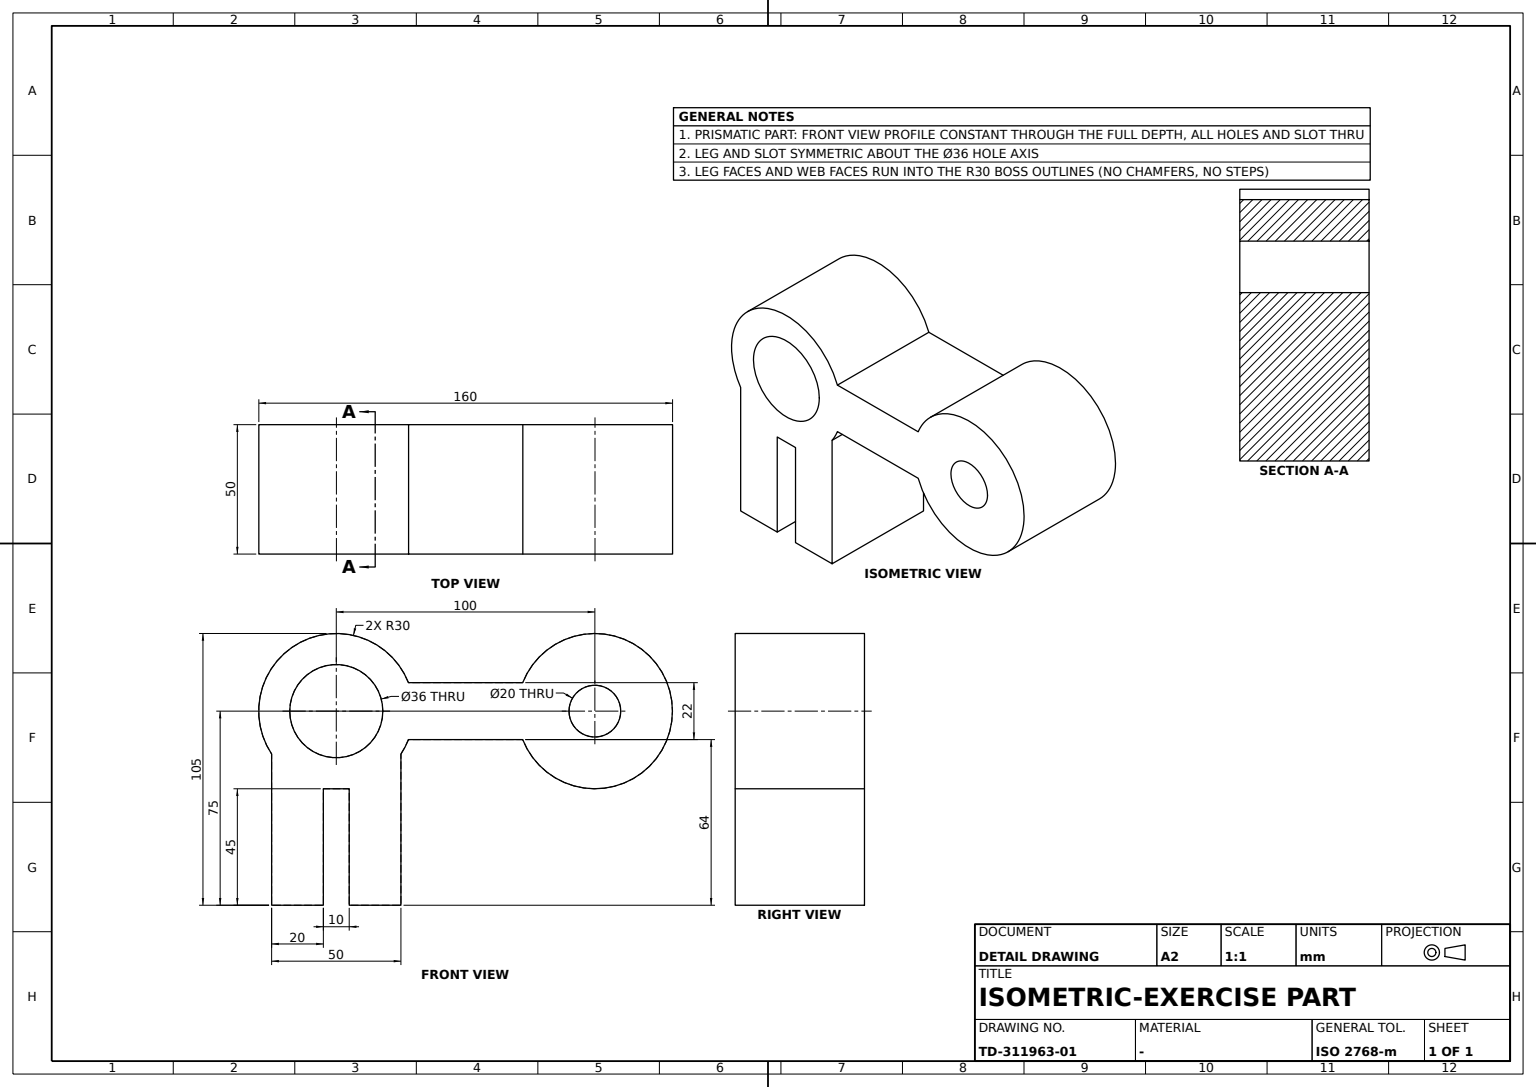
ISO-10303-21;
HEADER;
FILE_DESCRIPTION((''),'2;1');
FILE_NAME('','',(''),(''),'','','');
FILE_SCHEMA(('AUTOMOTIVE_DESIGN'));
ENDSEC;
DATA;
#1=APPLICATION_CONTEXT('');
#2=PRODUCT_CONTEXT('',#1,'mechanical');
#3=PRODUCT('','','',(#2));
#4=PRODUCT_DEFINITION_FORMATION('','',#3);
#5=PRODUCT_DEFINITION_CONTEXT('',#1,'design');
#6=PRODUCT_DEFINITION('','',#4,#5);
#7=PRODUCT_DEFINITION_SHAPE('','',#6);
#8=(LENGTH_UNIT()NAMED_UNIT(*)SI_UNIT(.MILLI.,.METRE.));
#9=(NAMED_UNIT(*)PLANE_ANGLE_UNIT()SI_UNIT($,.RADIAN.));
#10=(NAMED_UNIT(*)SI_UNIT($,.STERADIAN.)SOLID_ANGLE_UNIT());
#11=UNCERTAINTY_MEASURE_WITH_UNIT(LENGTH_MEASURE(1.E-05),#8,'distance_accuracy_value','');
#12=(GEOMETRIC_REPRESENTATION_CONTEXT(3)GLOBAL_UNCERTAINTY_ASSIGNED_CONTEXT((#11))GLOBAL_UNIT_ASSIGNED_CONTEXT((#8,#9,#10))REPRESENTATION_CONTEXT('',''));
#13=CARTESIAN_POINT('',(-25.,-25.,-16.583124));
#14=VERTEX_POINT('',#13);
#15=CARTESIAN_POINT('',(25.,-25.,-16.583124));
#16=VERTEX_POINT('',#15);
#17=CARTESIAN_POINT('',(0.,-25.,-16.583124));
#18=DIRECTION('',(1.,0.,0.));
#19=VECTOR('',#18,1000.);
#20=LINE('',#17,#19);
#21=EDGE_CURVE('',#14,#16,#20,.T.);
#22=ORIENTED_EDGE('',*,*,#21,.T.);
#23=CARTESIAN_POINT('',(25.,27.910571,11.));
#24=VERTEX_POINT('',#23);
#25=CARTESIAN_POINT('',(25.,0.,0.));
#26=DIRECTION('',(0.,1.,0.));
#27=AXIS2_PLACEMENT_3D('',#25,#18,#26);
#28=CIRCLE('',#27,30.);
#29=EDGE_CURVE('',#24,#16,#28,.T.);
#30=ORIENTED_EDGE('',*,*,#29,.F.);
#31=CARTESIAN_POINT('',(-25.,27.910571,11.));
#32=VERTEX_POINT('',#31);
#33=CARTESIAN_POINT('',(0.,27.910571,11.));
#34=LINE('',#33,#19);
#35=EDGE_CURVE('',#32,#24,#34,.T.);
#36=ORIENTED_EDGE('',*,*,#35,.F.);
#37=CARTESIAN_POINT('',(-25.,0.,0.));
#38=AXIS2_PLACEMENT_3D('',#37,#18,#26);
#39=CIRCLE('',#38,30.);
#40=EDGE_CURVE('',#32,#14,#39,.T.);
#41=ORIENTED_EDGE('',*,*,#40,.T.);
#42=EDGE_LOOP('',(#22,#30,#36,#41));
#43=FACE_OUTER_BOUND('',#42,.T.);
#44=CARTESIAN_POINT('',(0.,0.,0.));
#45=DIRECTION('',(-1.,0.,0.));
#46=AXIS2_PLACEMENT_3D('',#44,#45,#26);
#47=CYLINDRICAL_SURFACE('',#46,30.);
#48=ADVANCED_FACE('',(#43),#47,.T.);
#49=CARTESIAN_POINT('',(-25.,-25.,-75.));
#50=VERTEX_POINT('',#49);
#51=CARTESIAN_POINT('',(25.,-25.,-75.));
#52=VERTEX_POINT('',#51);
#53=CARTESIAN_POINT('',(0.,-25.,-75.));
#54=LINE('',#53,#19);
#55=EDGE_CURVE('',#50,#52,#54,.T.);
#56=ORIENTED_EDGE('',*,*,#55,.F.);
#57=CARTESIAN_POINT('',(-25.,-5.,-75.));
#58=VERTEX_POINT('',#57);
#59=CARTESIAN_POINT('',(-25.,-15.,-75.));
#60=VECTOR('',#26,1000.);
#61=LINE('',#59,#60);
#62=EDGE_CURVE('',#50,#58,#61,.T.);
#63=ORIENTED_EDGE('',*,*,#62,.T.);
#64=CARTESIAN_POINT('',(25.,-5.,-75.));
#65=VERTEX_POINT('',#64);
#66=CARTESIAN_POINT('',(0.,-5.,-75.));
#67=LINE('',#66,#19);
#68=EDGE_CURVE('',#58,#65,#67,.T.);
#69=ORIENTED_EDGE('',*,*,#68,.T.);
#70=CARTESIAN_POINT('',(25.,-15.,-75.));
#71=LINE('',#70,#60);
#72=EDGE_CURVE('',#52,#65,#71,.T.);
#73=ORIENTED_EDGE('',*,*,#72,.F.);
#74=EDGE_LOOP('',(#56,#63,#69,#73));
#75=FACE_OUTER_BOUND('',#74,.T.);
#76=DIRECTION('',(0.,0.,-1.));
#77=AXIS2_PLACEMENT_3D('',#53,#76,#26);
#78=PLANE('',#77);
#79=ADVANCED_FACE('',(#75),#78,.T.);
#80=CARTESIAN_POINT('',(25.,25.,-75.));
#81=VERTEX_POINT('',#80);
#82=CARTESIAN_POINT('',(25.,25.,-16.583124));
#83=VERTEX_POINT('',#82);
#84=CARTESIAN_POINT('',(25.,25.,-45.791562));
#85=DIRECTION('',(0.,0.,1.));
#86=VECTOR('',#85,1000.);
#87=LINE('',#84,#86);
#88=EDGE_CURVE('',#81,#83,#87,.T.);
#89=ORIENTED_EDGE('',*,*,#88,.F.);
#90=CARTESIAN_POINT('',(-25.,25.,-75.));
#91=VERTEX_POINT('',#90);
#92=CARTESIAN_POINT('',(0.,25.,-75.));
#93=LINE('',#92,#19);
#94=EDGE_CURVE('',#91,#81,#93,.T.);
#95=ORIENTED_EDGE('',*,*,#94,.F.);
#96=CARTESIAN_POINT('',(-25.,25.,-16.583124));
#97=VERTEX_POINT('',#96);
#98=CARTESIAN_POINT('',(-25.,25.,-45.791562));
#99=LINE('',#98,#86);
#100=EDGE_CURVE('',#91,#97,#99,.T.);
#101=ORIENTED_EDGE('',*,*,#100,.T.);
#102=CARTESIAN_POINT('',(0.,25.,-16.583124));
#103=LINE('',#102,#19);
#104=EDGE_CURVE('',#97,#83,#103,.T.);
#105=ORIENTED_EDGE('',*,*,#104,.T.);
#106=EDGE_LOOP('',(#89,#95,#101,#105));
#107=FACE_OUTER_BOUND('',#106,.T.);
#108=AXIS2_PLACEMENT_3D('',#92,#26,#85);
#109=PLANE('',#108);
#110=ADVANCED_FACE('',(#107),#109,.T.);
#111=CARTESIAN_POINT('',(-25.,110.,0.));
#112=VERTEX_POINT('',#111);
#113=CARTESIAN_POINT('',(25.,110.,0.));
#114=VERTEX_POINT('',#113);
#115=CARTESIAN_POINT('',(0.,110.,0.));
#116=LINE('',#115,#19);
#117=EDGE_CURVE('',#112,#114,#116,.T.);
#118=ORIENTED_EDGE('',*,*,#117,.T.);
#119=CARTESIAN_POINT('',(25.,90.,0.));
#120=VERTEX_POINT('',#119);
#121=CARTESIAN_POINT('',(25.,100.,0.));
#122=AXIS2_PLACEMENT_3D('',#121,#18,#26);
#123=CIRCLE('',#122,10.);
#124=EDGE_CURVE('',#114,#120,#123,.T.);
#125=ORIENTED_EDGE('',*,*,#124,.T.);
#126=CARTESIAN_POINT('',(-25.,90.,0.));
#127=VERTEX_POINT('',#126);
#128=CARTESIAN_POINT('',(0.,90.,0.));
#129=LINE('',#128,#19);
#130=EDGE_CURVE('',#127,#120,#129,.T.);
#131=ORIENTED_EDGE('',*,*,#130,.F.);
#132=CARTESIAN_POINT('',(-25.,100.,0.));
#133=AXIS2_PLACEMENT_3D('',#132,#18,#26);
#134=CIRCLE('',#133,10.);
#135=EDGE_CURVE('',#112,#127,#134,.T.);
#136=ORIENTED_EDGE('',*,*,#135,.F.);
#137=EDGE_LOOP('',(#118,#125,#131,#136));
#138=FACE_OUTER_BOUND('',#137,.T.);
#139=CARTESIAN_POINT('',(0.,100.,0.));
#140=AXIS2_PLACEMENT_3D('',#139,#45,#26);
#141=CYLINDRICAL_SURFACE('',#140,10.);
#142=ADVANCED_FACE('',(#138),#141,.F.);
#143=CARTESIAN_POINT('',(-25.,27.910571,-11.));
#144=VERTEX_POINT('',#143);
#145=CARTESIAN_POINT('',(25.,27.910571,-11.));
#146=VERTEX_POINT('',#145);
#147=CARTESIAN_POINT('',(0.,27.910571,-11.));
#148=LINE('',#147,#19);
#149=EDGE_CURVE('',#144,#146,#148,.T.);
#150=ORIENTED_EDGE('',*,*,#149,.T.);
#151=EDGE_CURVE('',#83,#146,#28,.T.);
#152=ORIENTED_EDGE('',*,*,#151,.F.);
#153=ORIENTED_EDGE('',*,*,#104,.F.);
#154=EDGE_CURVE('',#97,#144,#39,.T.);
#155=ORIENTED_EDGE('',*,*,#154,.T.);
#156=EDGE_LOOP('',(#150,#152,#153,#155));
#157=FACE_OUTER_BOUND('',#156,.T.);
#158=ADVANCED_FACE('',(#157),#47,.T.);
#159=CARTESIAN_POINT('',(25.,72.089429,11.));
#160=VERTEX_POINT('',#159);
#161=CARTESIAN_POINT('',(25.,50.,11.));
#162=DIRECTION('',(0.,-1.,0.));
#163=VECTOR('',#162,1000.);
#164=LINE('',#161,#163);
#165=EDGE_CURVE('',#160,#24,#164,.T.);
#166=ORIENTED_EDGE('',*,*,#165,.F.);
#167=CARTESIAN_POINT('',(-25.,72.089429,11.));
#168=VERTEX_POINT('',#167);
#169=CARTESIAN_POINT('',(0.,72.089429,11.));
#170=LINE('',#169,#19);
#171=EDGE_CURVE('',#168,#160,#170,.T.);
#172=ORIENTED_EDGE('',*,*,#171,.F.);
#173=CARTESIAN_POINT('',(-25.,50.,11.));
#174=LINE('',#173,#163);
#175=EDGE_CURVE('',#168,#32,#174,.T.);
#176=ORIENTED_EDGE('',*,*,#175,.T.);
#177=ORIENTED_EDGE('',*,*,#35,.T.);
#178=EDGE_LOOP('',(#166,#172,#176,#177));
#179=FACE_OUTER_BOUND('',#178,.T.);
#180=AXIS2_PLACEMENT_3D('',#33,#76,#26);
#181=PLANE('',#180);
#182=ADVANCED_FACE('',(#179),#181,.F.);
#183=CARTESIAN_POINT('',(-25.,-5.,-30.));
#184=VERTEX_POINT('',#183);
#185=CARTESIAN_POINT('',(-25.,-5.,-52.5));
#186=LINE('',#185,#86);
#187=EDGE_CURVE('',#58,#184,#186,.T.);
#188=ORIENTED_EDGE('',*,*,#187,.T.);
#189=CARTESIAN_POINT('',(25.,-5.,-30.));
#190=VERTEX_POINT('',#189);
#191=CARTESIAN_POINT('',(0.,-5.,-30.));
#192=LINE('',#191,#19);
#193=EDGE_CURVE('',#184,#190,#192,.T.);
#194=ORIENTED_EDGE('',*,*,#193,.T.);
#195=CARTESIAN_POINT('',(25.,-5.,-52.5));
#196=LINE('',#195,#86);
#197=EDGE_CURVE('',#65,#190,#196,.T.);
#198=ORIENTED_EDGE('',*,*,#197,.F.);
#199=ORIENTED_EDGE('',*,*,#68,.F.);
#200=EDGE_LOOP('',(#188,#194,#198,#199));
#201=FACE_OUTER_BOUND('',#200,.T.);
#202=AXIS2_PLACEMENT_3D('',#191,#162,#76);
#203=PLANE('',#202);
#204=ADVANCED_FACE('',(#201),#203,.F.);
#205=CARTESIAN_POINT('',(-25.,72.089429,-11.));
#206=VERTEX_POINT('',#205);
#207=CARTESIAN_POINT('',(-25.,50.,-11.));
#208=LINE('',#207,#60);
#209=EDGE_CURVE('',#144,#206,#208,.T.);
#210=ORIENTED_EDGE('',*,*,#209,.T.);
#211=CARTESIAN_POINT('',(25.,72.089429,-11.));
#212=VERTEX_POINT('',#211);
#213=CARTESIAN_POINT('',(0.,72.089429,-11.));
#214=LINE('',#213,#19);
#215=EDGE_CURVE('',#206,#212,#214,.T.);
#216=ORIENTED_EDGE('',*,*,#215,.T.);
#217=CARTESIAN_POINT('',(25.,50.,-11.));
#218=LINE('',#217,#60);
#219=EDGE_CURVE('',#146,#212,#218,.T.);
#220=ORIENTED_EDGE('',*,*,#219,.F.);
#221=ORIENTED_EDGE('',*,*,#149,.F.);
#222=EDGE_LOOP('',(#210,#216,#220,#221));
#223=FACE_OUTER_BOUND('',#222,.T.);
#224=AXIS2_PLACEMENT_3D('',#147,#76,#26);
#225=PLANE('',#224);
#226=ADVANCED_FACE('',(#223),#225,.T.);
#227=ORIENTED_EDGE('',*,*,#209,.F.);
#228=ORIENTED_EDGE('',*,*,#154,.F.);
#229=ORIENTED_EDGE('',*,*,#100,.F.);
#230=CARTESIAN_POINT('',(-25.,5.,-75.));
#231=VERTEX_POINT('',#230);
#232=CARTESIAN_POINT('',(-25.,15.,-75.));
#233=LINE('',#232,#60);
#234=EDGE_CURVE('',#231,#91,#233,.T.);
#235=ORIENTED_EDGE('',*,*,#234,.F.);
#236=CARTESIAN_POINT('',(-25.,5.,-30.));
#237=VERTEX_POINT('',#236);
#238=CARTESIAN_POINT('',(-25.,5.,-52.5));
#239=VECTOR('',#76,1000.);
#240=LINE('',#238,#239);
#241=EDGE_CURVE('',#237,#231,#240,.T.);
#242=ORIENTED_EDGE('',*,*,#241,.F.);
#243=CARTESIAN_POINT('',(-25.,0.,-30.));
#244=LINE('',#243,#60);
#245=EDGE_CURVE('',#184,#237,#244,.T.);
#246=ORIENTED_EDGE('',*,*,#245,.F.);
#247=ORIENTED_EDGE('',*,*,#187,.F.);
#248=ORIENTED_EDGE('',*,*,#62,.F.);
#249=CARTESIAN_POINT('',(-25.,-25.,-45.791562));
#250=LINE('',#249,#239);
#251=EDGE_CURVE('',#14,#50,#250,.T.);
#252=ORIENTED_EDGE('',*,*,#251,.F.);
#253=ORIENTED_EDGE('',*,*,#40,.F.);
#254=ORIENTED_EDGE('',*,*,#175,.F.);
#255=CARTESIAN_POINT('',(-25.,130.,0.));
#256=VERTEX_POINT('',#255);
#257=CIRCLE('',#133,30.);
#258=EDGE_CURVE('',#256,#168,#257,.T.);
#259=ORIENTED_EDGE('',*,*,#258,.F.);
#260=EDGE_CURVE('',#206,#256,#257,.T.);
#261=ORIENTED_EDGE('',*,*,#260,.F.);
#262=EDGE_LOOP('',(#227,#228,#229,#235,#242,#246,#247,#248,#252,#253,#254,#259,#261));
#263=FACE_OUTER_BOUND('',#262,.T.);
#264=CARTESIAN_POINT('',(-25.,-18.,0.));
#265=VERTEX_POINT('',#264);
#266=CARTESIAN_POINT('',(-25.,18.,0.));
#267=VERTEX_POINT('',#266);
#268=CIRCLE('',#38,18.);
#269=EDGE_CURVE('',#265,#267,#268,.T.);
#270=ORIENTED_EDGE('',*,*,#269,.T.);
#271=EDGE_CURVE('',#267,#265,#268,.T.);
#272=ORIENTED_EDGE('',*,*,#271,.T.);
#273=EDGE_LOOP('',(#270,#272));
#274=FACE_BOUND('',#273,.T.);
#275=EDGE_CURVE('',#127,#112,#134,.T.);
#276=ORIENTED_EDGE('',*,*,#275,.T.);
#277=ORIENTED_EDGE('',*,*,#135,.T.);
#278=EDGE_LOOP('',(#276,#277));
#279=FACE_BOUND('',#278,.T.);
#280=PLANE('',#38);
#281=ADVANCED_FACE('',(#263,#274,#279),#280,.F.);
#282=CARTESIAN_POINT('',(25.,5.,-75.));
#283=VERTEX_POINT('',#282);
#284=CARTESIAN_POINT('',(25.,15.,-75.));
#285=LINE('',#284,#60);
#286=EDGE_CURVE('',#283,#81,#285,.T.);
#287=ORIENTED_EDGE('',*,*,#286,.F.);
#288=CARTESIAN_POINT('',(0.,5.,-75.));
#289=LINE('',#288,#19);
#290=EDGE_CURVE('',#231,#283,#289,.T.);
#291=ORIENTED_EDGE('',*,*,#290,.F.);
#292=ORIENTED_EDGE('',*,*,#234,.T.);
#293=ORIENTED_EDGE('',*,*,#94,.T.);
#294=EDGE_LOOP('',(#287,#291,#292,#293));
#295=FACE_OUTER_BOUND('',#294,.T.);
#296=ADVANCED_FACE('',(#295),#78,.T.);
#297=ORIENTED_EDGE('',*,*,#251,.T.);
#298=ORIENTED_EDGE('',*,*,#55,.T.);
#299=CARTESIAN_POINT('',(25.,-25.,-45.791562));
#300=LINE('',#299,#239);
#301=EDGE_CURVE('',#16,#52,#300,.T.);
#302=ORIENTED_EDGE('',*,*,#301,.F.);
#303=ORIENTED_EDGE('',*,*,#21,.F.);
#304=EDGE_LOOP('',(#297,#298,#302,#303));
#305=FACE_OUTER_BOUND('',#304,.T.);
#306=AXIS2_PLACEMENT_3D('',#53,#26,#85);
#307=PLANE('',#306);
#308=ADVANCED_FACE('',(#305),#307,.F.);
#309=ORIENTED_EDGE('',*,*,#193,.F.);
#310=ORIENTED_EDGE('',*,*,#245,.T.);
#311=CARTESIAN_POINT('',(25.,5.,-30.));
#312=VERTEX_POINT('',#311);
#313=CARTESIAN_POINT('',(0.,5.,-30.));
#314=LINE('',#313,#19);
#315=EDGE_CURVE('',#237,#312,#314,.T.);
#316=ORIENTED_EDGE('',*,*,#315,.T.);
#317=CARTESIAN_POINT('',(25.,0.,-30.));
#318=LINE('',#317,#60);
#319=EDGE_CURVE('',#190,#312,#318,.T.);
#320=ORIENTED_EDGE('',*,*,#319,.F.);
#321=EDGE_LOOP('',(#309,#310,#316,#320));
#322=FACE_OUTER_BOUND('',#321,.T.);
#323=AXIS2_PLACEMENT_3D('',#313,#85,#162);
#324=PLANE('',#323);
#325=ADVANCED_FACE('',(#322),#324,.F.);
#326=CARTESIAN_POINT('',(25.,18.,0.));
#327=VERTEX_POINT('',#326);
#328=CARTESIAN_POINT('',(0.,18.,0.));
#329=LINE('',#328,#19);
#330=EDGE_CURVE('',#267,#327,#329,.T.);
#331=ORIENTED_EDGE('',*,*,#330,.F.);
#332=ORIENTED_EDGE('',*,*,#269,.F.);
#333=CARTESIAN_POINT('',(25.,-18.,0.));
#334=VERTEX_POINT('',#333);
#335=CARTESIAN_POINT('',(0.,-18.,0.));
#336=LINE('',#335,#19);
#337=EDGE_CURVE('',#265,#334,#336,.T.);
#338=ORIENTED_EDGE('',*,*,#337,.T.);
#339=CIRCLE('',#27,18.);
#340=EDGE_CURVE('',#334,#327,#339,.T.);
#341=ORIENTED_EDGE('',*,*,#340,.T.);
#342=EDGE_LOOP('',(#331,#332,#338,#341));
#343=FACE_OUTER_BOUND('',#342,.T.);
#344=CYLINDRICAL_SURFACE('',#46,18.);
#345=ADVANCED_FACE('',(#343),#344,.F.);
#346=CARTESIAN_POINT('',(25.,5.,-52.5));
#347=LINE('',#346,#239);
#348=EDGE_CURVE('',#312,#283,#347,.T.);
#349=ORIENTED_EDGE('',*,*,#348,.F.);
#350=ORIENTED_EDGE('',*,*,#315,.F.);
#351=ORIENTED_EDGE('',*,*,#241,.T.);
#352=ORIENTED_EDGE('',*,*,#290,.T.);
#353=EDGE_LOOP('',(#349,#350,#351,#352));
#354=FACE_OUTER_BOUND('',#353,.T.);
#355=AXIS2_PLACEMENT_3D('',#313,#162,#76);
#356=PLANE('',#355);
#357=ADVANCED_FACE('',(#354),#356,.T.);
#358=CARTESIAN_POINT('',(25.,130.,0.));
#359=VERTEX_POINT('',#358);
#360=CARTESIAN_POINT('',(0.,130.,0.));
#361=LINE('',#360,#19);
#362=EDGE_CURVE('',#256,#359,#361,.T.);
#363=ORIENTED_EDGE('',*,*,#362,.T.);
#364=CIRCLE('',#122,30.);
#365=EDGE_CURVE('',#212,#359,#364,.T.);
#366=ORIENTED_EDGE('',*,*,#365,.F.);
#367=ORIENTED_EDGE('',*,*,#215,.F.);
#368=ORIENTED_EDGE('',*,*,#260,.T.);
#369=EDGE_LOOP('',(#363,#366,#367,#368));
#370=FACE_OUTER_BOUND('',#369,.T.);
#371=CYLINDRICAL_SURFACE('',#140,30.);
#372=ADVANCED_FACE('',(#370),#371,.T.);
#373=ORIENTED_EDGE('',*,*,#117,.F.);
#374=ORIENTED_EDGE('',*,*,#275,.F.);
#375=ORIENTED_EDGE('',*,*,#130,.T.);
#376=EDGE_CURVE('',#120,#114,#123,.T.);
#377=ORIENTED_EDGE('',*,*,#376,.T.);
#378=EDGE_LOOP('',(#373,#374,#375,#377));
#379=FACE_OUTER_BOUND('',#378,.T.);
#380=ADVANCED_FACE('',(#379),#141,.F.);
#381=ORIENTED_EDGE('',*,*,#340,.F.);
#382=EDGE_CURVE('',#327,#334,#339,.T.);
#383=ORIENTED_EDGE('',*,*,#382,.F.);
#384=EDGE_LOOP('',(#381,#383));
#385=FACE_BOUND('',#384,.T.);
#386=ORIENTED_EDGE('',*,*,#197,.T.);
#387=ORIENTED_EDGE('',*,*,#319,.T.);
#388=ORIENTED_EDGE('',*,*,#348,.T.);
#389=ORIENTED_EDGE('',*,*,#286,.T.);
#390=ORIENTED_EDGE('',*,*,#88,.T.);
#391=ORIENTED_EDGE('',*,*,#151,.T.);
#392=ORIENTED_EDGE('',*,*,#219,.T.);
#393=ORIENTED_EDGE('',*,*,#365,.T.);
#394=EDGE_CURVE('',#359,#160,#364,.T.);
#395=ORIENTED_EDGE('',*,*,#394,.T.);
#396=ORIENTED_EDGE('',*,*,#165,.T.);
#397=ORIENTED_EDGE('',*,*,#29,.T.);
#398=ORIENTED_EDGE('',*,*,#301,.T.);
#399=ORIENTED_EDGE('',*,*,#72,.T.);
#400=EDGE_LOOP('',(#386,#387,#388,#389,#390,#391,#392,#393,#395,#396,#397,#398,#399));
#401=FACE_OUTER_BOUND('',#400,.T.);
#402=ORIENTED_EDGE('',*,*,#376,.F.);
#403=ORIENTED_EDGE('',*,*,#124,.F.);
#404=EDGE_LOOP('',(#402,#403));
#405=FACE_BOUND('',#404,.T.);
#406=PLANE('',#27);
#407=ADVANCED_FACE('',(#385,#401,#405),#406,.T.);
#408=ORIENTED_EDGE('',*,*,#271,.F.);
#409=ORIENTED_EDGE('',*,*,#330,.T.);
#410=ORIENTED_EDGE('',*,*,#382,.T.);
#411=ORIENTED_EDGE('',*,*,#337,.F.);
#412=EDGE_LOOP('',(#408,#409,#410,#411));
#413=FACE_OUTER_BOUND('',#412,.T.);
#414=ADVANCED_FACE('',(#413),#344,.F.);
#415=ORIENTED_EDGE('',*,*,#362,.F.);
#416=ORIENTED_EDGE('',*,*,#258,.T.);
#417=ORIENTED_EDGE('',*,*,#171,.T.);
#418=ORIENTED_EDGE('',*,*,#394,.F.);
#419=EDGE_LOOP('',(#415,#416,#417,#418));
#420=FACE_OUTER_BOUND('',#419,.T.);
#421=ADVANCED_FACE('',(#420),#371,.T.);
#422=CLOSED_SHELL('',(#48,#79,#110,#142,#158,#182,#204,#226,#281,#296,#308,#325,#345,#357,#372,#380,#407,#414,#421));
#423=MANIFOLD_SOLID_BREP('',#422);
#424=ADVANCED_BREP_SHAPE_REPRESENTATION('',(#423),#12);
#425=SHAPE_DEFINITION_REPRESENTATION(#7,#424);
ENDSEC;
END-ISO-10303-21;
